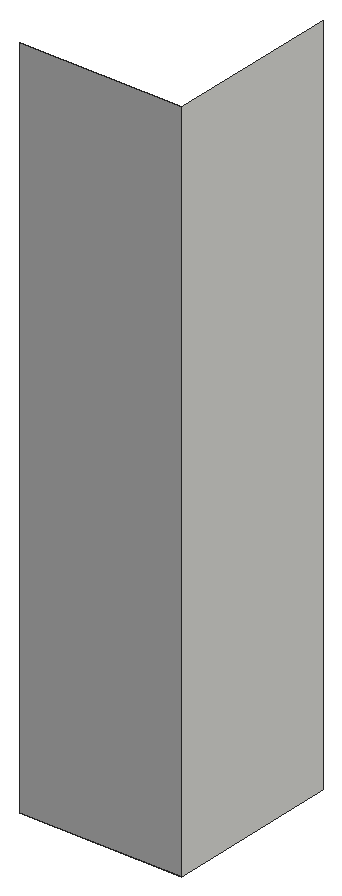
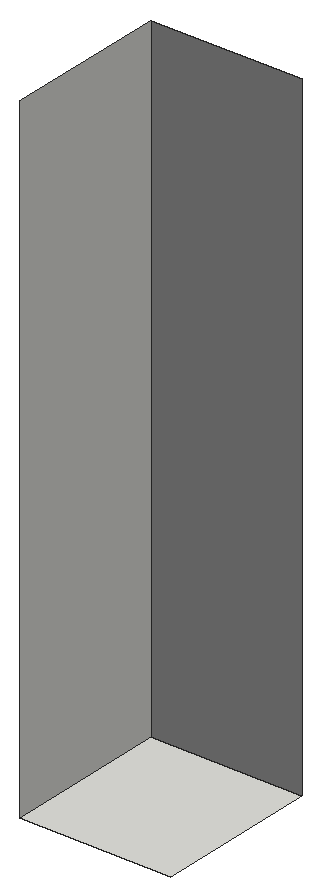
# SketchUp Ruby script. Lengths in inches.
U = 1.inch
M = Sketchup.active_model
def pt(a) = Geom::Point3d.new(a.map { |v| v * U })
def face(e, loops, mat)
  f = e.add_face(loops[0].map { |a| pt(a) })
  loops[1..].each { |l| e.add_face(l.map { |a| pt(a) }).erase! }
  f.material = f.back_material = mat if mat
  f
end
# faces: each face lists its corners as indices into pts; further lists are holes
def faces(e, pts, list, mat = nil) = list.each { |f| face(e, (f[0].is_a?(Array) ? f : [f]).map { |l| l.map { |i| pts[i] } }, mat) }
# xy, xz, yz: faces in a plane at the given z, y or x. An outline is a flat list of corners, or four numbers for a rectangle; further outlines are holes
def ring(l) = l.size == 4 ? [[l[0], l[1]], [l[2], l[1]], [l[2], l[3]], [l[0], l[3]]] : l.each_slice(2).to_a
def flat(e, list, mat, &to3) = list.each { |f| face(e, (f[0].is_a?(Array) ? f : [f]).map { |l| ring(l).map { |u, v| to3.(u, v) } }, mat) }
def xy(e, z, list, mat = nil) = flat(e, list, mat) { |x, y| [x, y, z] }
def xz(e, y, list, mat = nil) = flat(e, list, mat) { |x, z| [x, y, z] }
def yz(e, x, list, mat = nil) = flat(e, list, mat) { |y, z| [x, y, z] }
def lines(e, pts, list) = list.each { |a, b| e.add_line(pt(pts[a]), pt(pts[b])) }
# prism: a flat outline (further loops are holes) pulled along v
def prism(e, loops, v, mat = nil)
  f = face(e, loops, mat); d = Geom::Vector3d.new(v.map { |x| x * U })
  f.pushpull(f.normal.samedirection?(d) ? d.length : -d.length)
end
def box(e, o, s, mat = nil) = prism(e, [[o, [o[0] + s[0], o[1], o[2]], [o[0] + s[0], o[1] + s[1], o[2]], [o[0], o[1] + s[1], o[2]]]], [0, 0, s[2]], mat)
def at(x, y, z, deg = 0) = Geom::Transformation.translation(pt([x, y, z])) * Geom::Transformation.rotation(ORIGIN, Z_AXIS, deg.degrees)
def axes(o, x, y, z) = Geom::Transformation.new([*x, 0, *y, 0, *z, 0, *pt(o).to_a, 1])
def part(name) = M.definitions.add(name)
# library, detail: a bought-in or finely detailed component or shape, given as its bounding box
def library(name, o, s) = part(name).tap { |d| box(d.entities, o, s) }
def detail(e, o, s) = box(e.add_group.entities, o, s)
def put(e, d, t, mat = nil) = e.add_instance(d, t).tap { |i| i.material = mat if mat }
def group(e, t, mat = nil) = e.add_group.tap { |g| g.transformation = t; g.material = mat if mat }.entities
root = M.entities
M.materials.add("[Blinds Vertical Stripe Gray]").color = [160, 160, 160]
xy(root,0,[[192.64,96.24,206.19,111]])
xz(root,96.24,[[192.64,0,206.19,57.8125]],"[Blinds Vertical Stripe Gray]")
yz(root,206.19,[[96.24,0,111,57.8125]])
